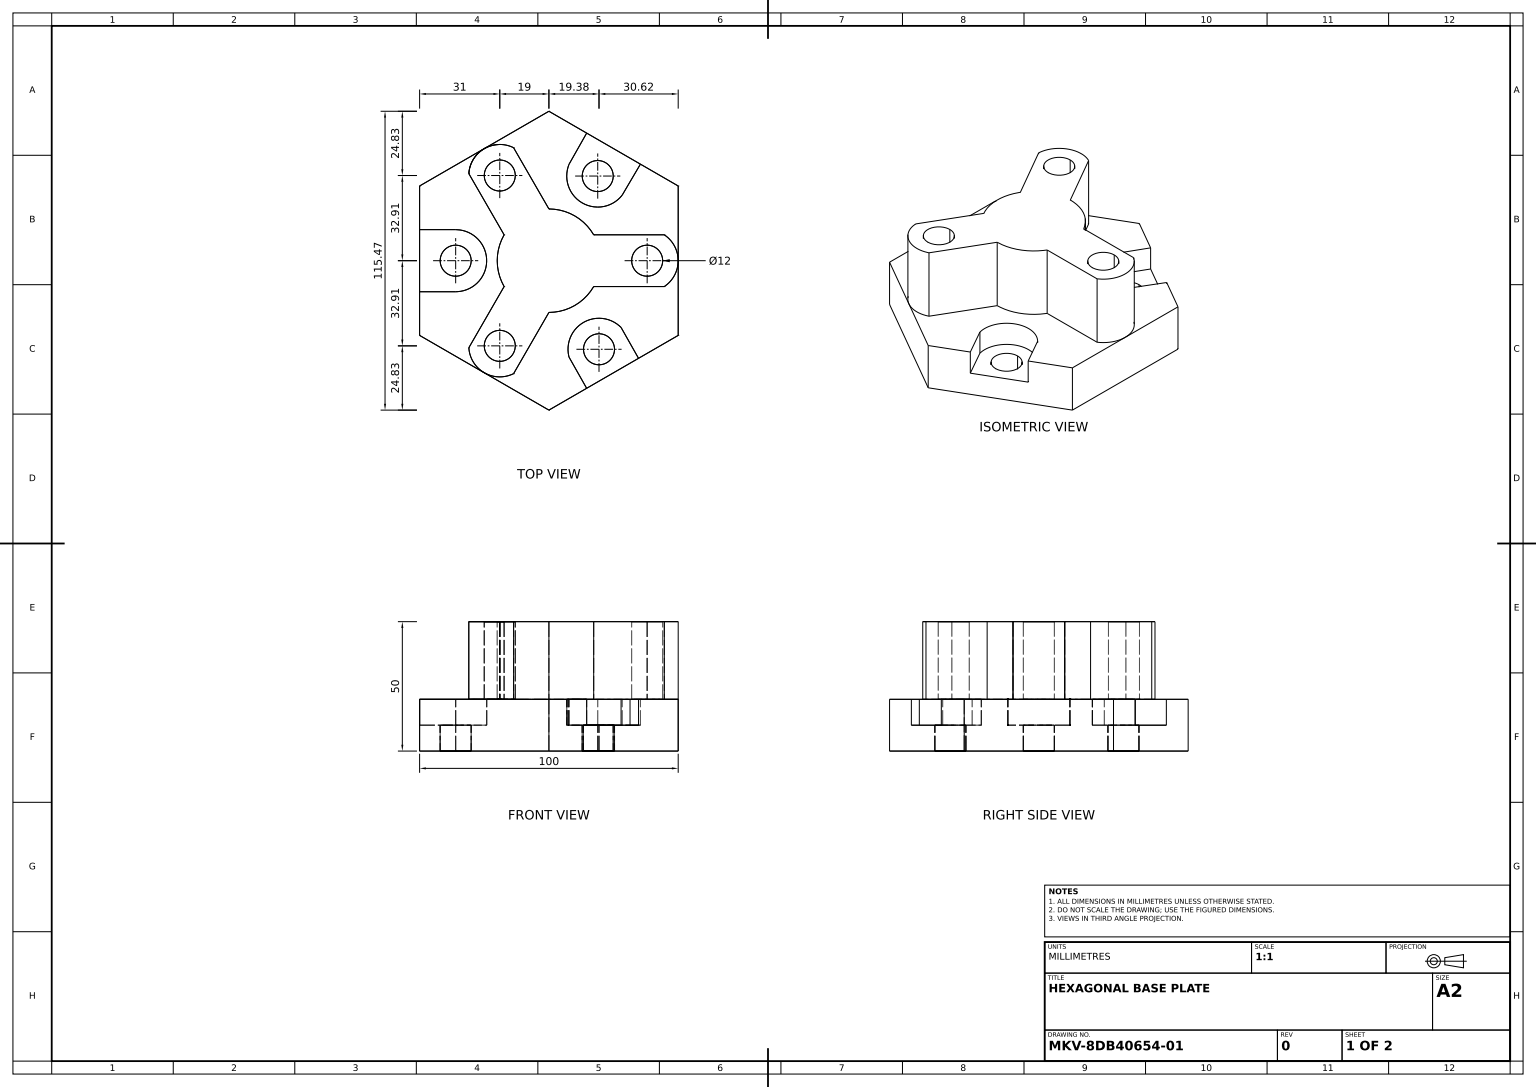
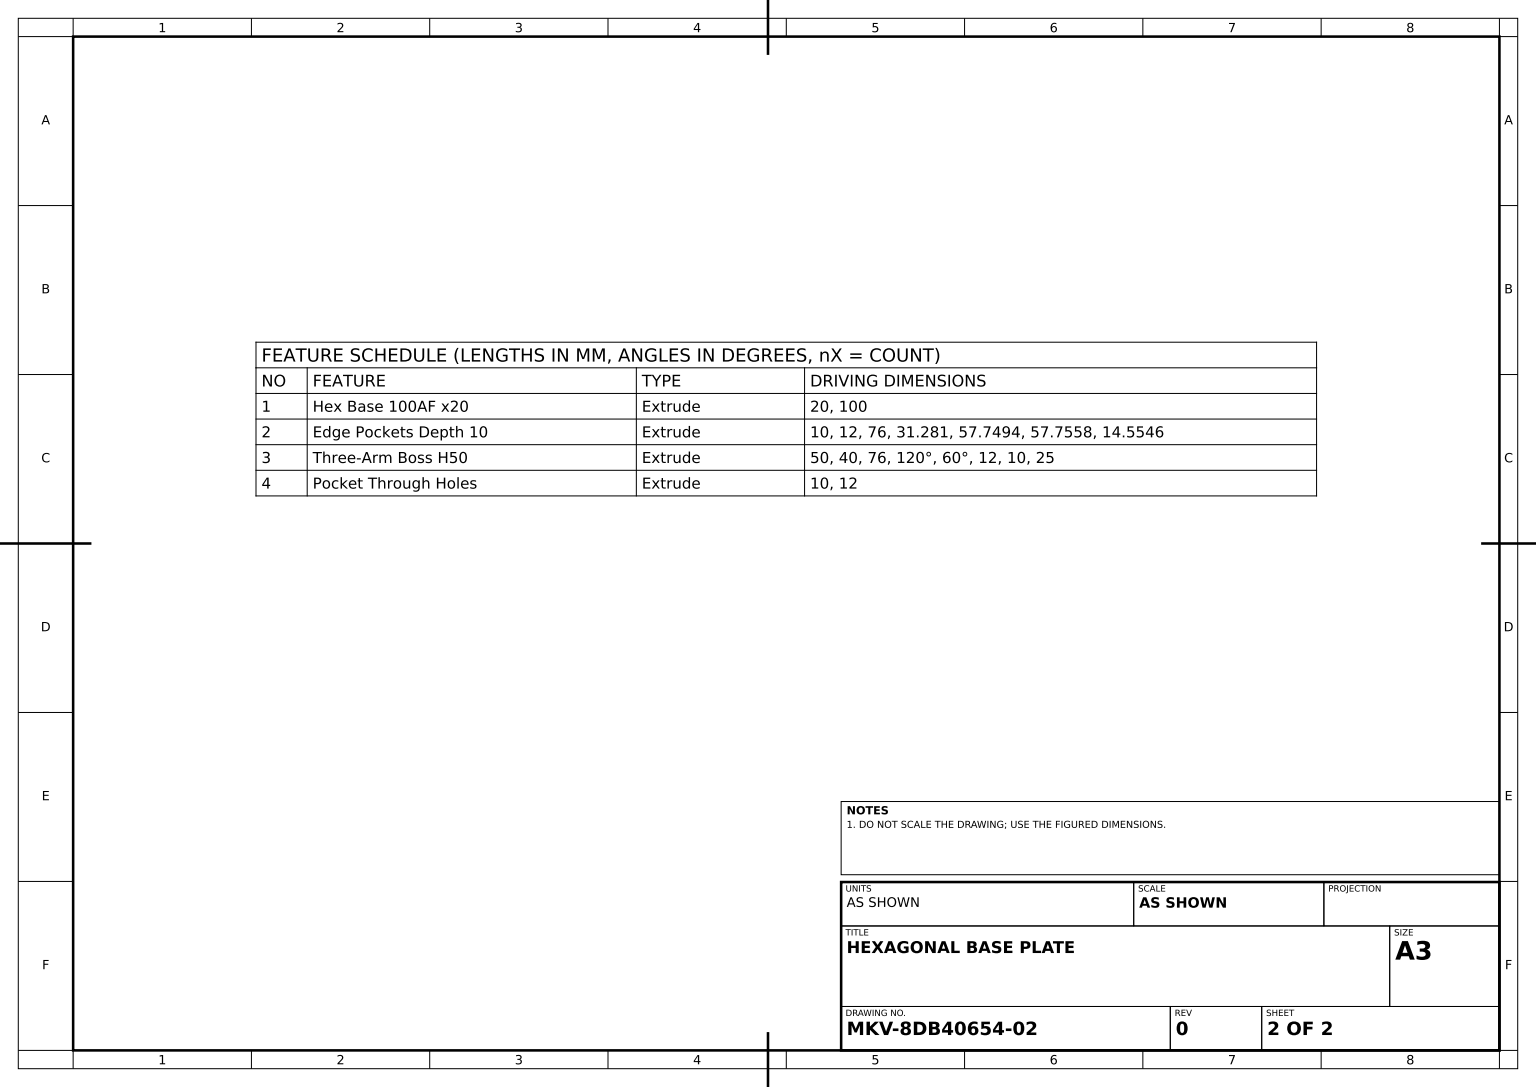
ISO-10303-21;
HEADER;
FILE_DESCRIPTION((''),'2;1');
FILE_NAME('','',(''),(''),'','','');
FILE_SCHEMA(('AUTOMOTIVE_DESIGN'));
ENDSEC;
DATA;
#1=APPLICATION_CONTEXT('');
#2=PRODUCT_CONTEXT('',#1,'mechanical');
#3=PRODUCT('','','',(#2));
#4=PRODUCT_DEFINITION_FORMATION('','',#3);
#5=PRODUCT_DEFINITION_CONTEXT('',#1,'design');
#6=PRODUCT_DEFINITION('','',#4,#5);
#7=PRODUCT_DEFINITION_SHAPE('','',#6);
#8=(LENGTH_UNIT()NAMED_UNIT(*)SI_UNIT(.MILLI.,.METRE.));
#9=(NAMED_UNIT(*)PLANE_ANGLE_UNIT()SI_UNIT($,.RADIAN.));
#10=(NAMED_UNIT(*)SI_UNIT($,.STERADIAN.)SOLID_ANGLE_UNIT());
#11=UNCERTAINTY_MEASURE_WITH_UNIT(LENGTH_MEASURE(1.E-05),#8,'distance_accuracy_value','');
#12=(GEOMETRIC_REPRESENTATION_CONTEXT(3)GLOBAL_UNCERTAINTY_ASSIGNED_CONTEXT((#11))GLOBAL_UNIT_ASSIGNED_CONTEXT((#8,#9,#10))REPRESENTATION_CONTEXT('',''));
#13=CARTESIAN_POINT('',(-50.,10.,-12.));
#14=VERTEX_POINT('',#13);
#15=CARTESIAN_POINT('',(-50.,20.,-12.));
#16=VERTEX_POINT('',#15);
#17=DIRECTION('',(0.,1.,0.));
#18=VECTOR('',#17,1000.);
#19=LINE('',#13,#18);
#20=EDGE_CURVE('',#14,#16,#19,.T.);
#21=ORIENTED_EDGE('',*,*,#20,.F.);
#22=CARTESIAN_POINT('',(-36.055514,10.,-12.));
#23=VERTEX_POINT('',#22);
#24=CARTESIAN_POINT('',(0.,10.,-12.));
#25=DIRECTION('',(1.,0.,0.));
#26=VECTOR('',#25,1000.);
#27=LINE('',#24,#26);
#28=EDGE_CURVE('',#14,#23,#27,.T.);
#29=ORIENTED_EDGE('',*,*,#28,.T.);
#30=CARTESIAN_POINT('',(-36.055514,20.,-12.));
#31=VERTEX_POINT('',#30);
#32=LINE('',#22,#18);
#33=EDGE_CURVE('',#23,#31,#32,.T.);
#34=ORIENTED_EDGE('',*,*,#33,.T.);
#35=CARTESIAN_POINT('',(0.,20.,-12.));
#36=LINE('',#35,#26);
#37=EDGE_CURVE('',#16,#31,#36,.T.);
#38=ORIENTED_EDGE('',*,*,#37,.F.);
#39=EDGE_LOOP('',(#21,#29,#34,#38));
#40=FACE_OUTER_BOUND('',#39,.T.);
#41=DIRECTION('',(0.,0.,1.));
#42=AXIS2_PLACEMENT_3D('',#24,#41,#25);
#43=PLANE('',#42);
#44=ADVANCED_FACE('',(#40),#43,.T.);
#45=CARTESIAN_POINT('',(18.881704,0.,-38.704071));
#46=VERTEX_POINT('',#45);
#47=CARTESIAN_POINT('',(18.881704,10.,-38.704071));
#48=VERTEX_POINT('',#47);
#49=LINE('',#45,#18);
#50=EDGE_CURVE('',#46,#48,#49,.T.);
#51=ORIENTED_EDGE('',*,*,#50,.F.);
#52=CARTESIAN_POINT('',(18.881704,0.,-26.704071));
#53=VERTEX_POINT('',#52);
#54=CARTESIAN_POINT('',(18.881704,0.,-32.704071));
#55=AXIS2_PLACEMENT_3D('',#54,#17,#41);
#56=CIRCLE('',#55,6.);
#57=EDGE_CURVE('',#53,#46,#56,.T.);
#58=ORIENTED_EDGE('',*,*,#57,.F.);
#59=CARTESIAN_POINT('',(18.881704,10.,-26.704071));
#60=VERTEX_POINT('',#59);
#61=LINE('',#52,#18);
#62=EDGE_CURVE('',#53,#60,#61,.T.);
#63=ORIENTED_EDGE('',*,*,#62,.T.);
#64=CARTESIAN_POINT('',(18.881704,10.,-32.704071));
#65=AXIS2_PLACEMENT_3D('',#64,#17,#41);
#66=CIRCLE('',#65,6.);
#67=EDGE_CURVE('',#60,#48,#66,.T.);
#68=ORIENTED_EDGE('',*,*,#67,.T.);
#69=EDGE_LOOP('',(#51,#58,#63,#68));
#70=FACE_OUTER_BOUND('',#69,.T.);
#71=CYLINDRICAL_SURFACE('',#55,6.);
#72=ADVANCED_FACE('',(#70),#71,.F.);
#73=CARTESIAN_POINT('',(50.,20.,0.));
#74=VERTEX_POINT('',#73);
#75=CARTESIAN_POINT('',(44.63325,20.,10.));
#76=VERTEX_POINT('',#75);
#77=CARTESIAN_POINT('',(38.,20.,0.));
#78=DIRECTION('',(0.,-1.,0.));
#79=AXIS2_PLACEMENT_3D('',#77,#78,#41);
#80=CIRCLE('',#79,12.);
#81=EDGE_CURVE('',#74,#76,#80,.T.);
#82=ORIENTED_EDGE('',*,*,#81,.F.);
#83=CARTESIAN_POINT('',(44.63325,20.,-10.));
#84=VERTEX_POINT('',#83);
#85=EDGE_CURVE('',#84,#74,#80,.T.);
#86=ORIENTED_EDGE('',*,*,#85,.F.);
#87=CARTESIAN_POINT('',(44.63325,50.,-10.));
#88=VERTEX_POINT('',#87);
#89=VECTOR('',#78,1000.);
#90=LINE('',#87,#89);
#91=EDGE_CURVE('',#88,#84,#90,.T.);
#92=ORIENTED_EDGE('',*,*,#91,.F.);
#93=CARTESIAN_POINT('',(44.63325,50.,10.));
#94=VERTEX_POINT('',#93);
#95=CARTESIAN_POINT('',(38.,50.,0.));
#96=AXIS2_PLACEMENT_3D('',#95,#17,#41);
#97=CIRCLE('',#96,12.);
#98=EDGE_CURVE('',#94,#88,#97,.T.);
#99=ORIENTED_EDGE('',*,*,#98,.F.);
#100=LINE('',#93,#89);
#101=EDGE_CURVE('',#94,#76,#100,.T.);
#102=ORIENTED_EDGE('',*,*,#101,.T.);
#103=EDGE_LOOP('',(#82,#86,#92,#99,#102));
#104=FACE_OUTER_BOUND('',#103,.T.);
#105=DIRECTION('',(0.,0.,-1.));
#106=AXIS2_PLACEMENT_3D('',#95,#78,#105);
#107=CYLINDRICAL_SURFACE('',#106,12.);
#108=ADVANCED_FACE('',(#104),#107,.T.);
#109=CARTESIAN_POINT('',(-36.055514,10.,12.));
#110=VERTEX_POINT('',#109);
#111=CARTESIAN_POINT('',(-36.055514,20.,12.));
#112=VERTEX_POINT('',#111);
#113=LINE('',#109,#18);
#114=EDGE_CURVE('',#110,#112,#113,.T.);
#115=ORIENTED_EDGE('',*,*,#114,.T.);
#116=CARTESIAN_POINT('',(-36.055514,20.,0.));
#117=AXIS2_PLACEMENT_3D('',#116,#78,#41);
#118=CIRCLE('',#117,12.);
#119=EDGE_CURVE('',#31,#112,#118,.T.);
#120=ORIENTED_EDGE('',*,*,#119,.F.);
#121=ORIENTED_EDGE('',*,*,#33,.F.);
#122=CARTESIAN_POINT('',(-36.055514,10.,0.));
#123=AXIS2_PLACEMENT_3D('',#122,#78,#41);
#124=CIRCLE('',#123,12.);
#125=EDGE_CURVE('',#23,#110,#124,.T.);
#126=ORIENTED_EDGE('',*,*,#125,.T.);
#127=EDGE_LOOP('',(#115,#120,#121,#126));
#128=FACE_OUTER_BOUND('',#127,.T.);
#129=AXIS2_PLACEMENT_3D('',#122,#17,#41);
#130=CYLINDRICAL_SURFACE('',#129,12.);
#131=ADVANCED_FACE('',(#128),#130,.F.);
#132=CARTESIAN_POINT('',(28.338333,20.,-25.316773));
#133=VERTEX_POINT('',#132);
#134=CARTESIAN_POINT('',(18.881704,20.,-20.704071));
#135=VERTEX_POINT('',#134);
#136=CARTESIAN_POINT('',(18.881704,20.,-32.704071));
#137=AXIS2_PLACEMENT_3D('',#136,#78,#41);
#138=CIRCLE('',#137,12.);
#139=EDGE_CURVE('',#133,#135,#138,.T.);
#140=ORIENTED_EDGE('',*,*,#139,.F.);
#141=CARTESIAN_POINT('',(28.338333,10.,-25.316773));
#142=VERTEX_POINT('',#141);
#143=LINE('',#141,#18);
#144=EDGE_CURVE('',#142,#133,#143,.T.);
#145=ORIENTED_EDGE('',*,*,#144,.F.);
#146=CARTESIAN_POINT('',(18.881704,10.,-20.704071));
#147=VERTEX_POINT('',#146);
#148=AXIS2_PLACEMENT_3D('',#64,#78,#41);
#149=CIRCLE('',#148,12.);
#150=EDGE_CURVE('',#142,#147,#149,.T.);
#151=ORIENTED_EDGE('',*,*,#150,.T.);
#152=LINE('',#146,#18);
#153=EDGE_CURVE('',#147,#135,#152,.T.);
#154=ORIENTED_EDGE('',*,*,#153,.T.);
#155=EDGE_LOOP('',(#140,#145,#151,#154));
#156=FACE_OUTER_BOUND('',#155,.T.);
#157=CYLINDRICAL_SURFACE('',#65,12.);
#158=ADVANCED_FACE('',(#156),#157,.F.);
#159=ORIENTED_EDGE('',*,*,#20,.T.);
#160=CARTESIAN_POINT('',(-50.,20.,-28.867513));
#161=VERTEX_POINT('',#160);
#162=VECTOR('',#41,1000.);
#163=LINE('',#160,#162);
#164=EDGE_CURVE('',#161,#16,#163,.T.);
#165=ORIENTED_EDGE('',*,*,#164,.F.);
#166=CARTESIAN_POINT('',(-50.,0.,-28.867513));
#167=VERTEX_POINT('',#166);
#168=LINE('',#160,#89);
#169=EDGE_CURVE('',#161,#167,#168,.T.);
#170=ORIENTED_EDGE('',*,*,#169,.T.);
#171=CARTESIAN_POINT('',(-50.,0.,28.867513));
#172=VERTEX_POINT('',#171);
#173=LINE('',#166,#162);
#174=EDGE_CURVE('',#167,#172,#173,.T.);
#175=ORIENTED_EDGE('',*,*,#174,.T.);
#176=CARTESIAN_POINT('',(-50.,20.,28.867513));
#177=VERTEX_POINT('',#176);
#178=LINE('',#176,#89);
#179=EDGE_CURVE('',#177,#172,#178,.T.);
#180=ORIENTED_EDGE('',*,*,#179,.F.);
#181=CARTESIAN_POINT('',(-50.,20.,12.));
#182=VERTEX_POINT('',#181);
#183=EDGE_CURVE('',#182,#177,#163,.T.);
#184=ORIENTED_EDGE('',*,*,#183,.F.);
#185=CARTESIAN_POINT('',(-50.,10.,12.));
#186=VERTEX_POINT('',#185);
#187=LINE('',#185,#18);
#188=EDGE_CURVE('',#186,#182,#187,.T.);
#189=ORIENTED_EDGE('',*,*,#188,.F.);
#190=CARTESIAN_POINT('',(-50.,10.,0.));
#191=LINE('',#190,#162);
#192=EDGE_CURVE('',#14,#186,#191,.T.);
#193=ORIENTED_EDGE('',*,*,#192,.F.);
#194=EDGE_LOOP('',(#159,#165,#170,#175,#180,#184,#189,#193));
#195=FACE_OUTER_BOUND('',#194,.T.);
#196=AXIS2_PLACEMENT_3D('',#160,#25,#105);
#197=PLANE('',#196);
#198=ADVANCED_FACE('',(#195),#197,.F.);
#199=CARTESIAN_POINT('',(-17.320508,50.,10.));
#200=VERTEX_POINT('',#199);
#201=CARTESIAN_POINT('',(-30.976879,50.,33.653528));
#202=VERTEX_POINT('',#201);
#203=CARTESIAN_POINT('',(-8.660254,50.,-5.));
#204=DIRECTION('',(-0.5,0.,0.866025404));
#205=VECTOR('',#204,1000.);
#206=LINE('',#203,#205);
#207=EDGE_CURVE('',#200,#202,#206,.T.);
#208=ORIENTED_EDGE('',*,*,#207,.T.);
#209=CARTESIAN_POINT('',(-13.656371,50.,43.653528));
#210=VERTEX_POINT('',#209);
#211=CARTESIAN_POINT('',(-19.,50.,32.908965));
#212=AXIS2_PLACEMENT_3D('',#211,#17,#41);
#213=CIRCLE('',#212,12.);
#214=EDGE_CURVE('',#202,#210,#213,.T.);
#215=ORIENTED_EDGE('',*,*,#214,.T.);
#216=CARTESIAN_POINT('',(0.,50.,20.));
#217=VERTEX_POINT('',#216);
#218=CARTESIAN_POINT('',(8.660254,50.,5.));
#219=LINE('',#218,#205);
#220=EDGE_CURVE('',#217,#210,#219,.T.);
#221=ORIENTED_EDGE('',*,*,#220,.F.);
#222=CARTESIAN_POINT('',(17.320508,50.,10.));
#223=VERTEX_POINT('',#222);
#224=CARTESIAN_POINT('',(0.,50.,0.));
#225=AXIS2_PLACEMENT_3D('',#224,#17,#41);
#226=CIRCLE('',#225,20.);
#227=EDGE_CURVE('',#217,#223,#226,.T.);
#228=ORIENTED_EDGE('',*,*,#227,.T.);
#229=CARTESIAN_POINT('',(0.,50.,10.));
#230=LINE('',#229,#26);
#231=EDGE_CURVE('',#223,#94,#230,.T.);
#232=ORIENTED_EDGE('',*,*,#231,.T.);
#233=ORIENTED_EDGE('',*,*,#98,.T.);
#234=CARTESIAN_POINT('',(17.320508,50.,-10.));
#235=VERTEX_POINT('',#234);
#236=CARTESIAN_POINT('',(0.,50.,-10.));
#237=LINE('',#236,#26);
#238=EDGE_CURVE('',#235,#88,#237,.T.);
#239=ORIENTED_EDGE('',*,*,#238,.F.);
#240=CARTESIAN_POINT('',(0.,50.,-20.));
#241=VERTEX_POINT('',#240);
#242=EDGE_CURVE('',#235,#241,#226,.T.);
#243=ORIENTED_EDGE('',*,*,#242,.T.);
#244=CARTESIAN_POINT('',(-13.656371,50.,-43.653528));
#245=VERTEX_POINT('',#244);
#246=CARTESIAN_POINT('',(8.660254,50.,-5.));
#247=DIRECTION('',(-0.5,0.,-0.866025404));
#248=VECTOR('',#247,1000.);
#249=LINE('',#246,#248);
#250=EDGE_CURVE('',#241,#245,#249,.T.);
#251=ORIENTED_EDGE('',*,*,#250,.T.);
#252=CARTESIAN_POINT('',(-19.,50.,-44.908965));
#253=VERTEX_POINT('',#252);
#254=CARTESIAN_POINT('',(-19.,50.,-32.908965));
#255=AXIS2_PLACEMENT_3D('',#254,#17,#41);
#256=CIRCLE('',#255,12.);
#257=EDGE_CURVE('',#245,#253,#256,.T.);
#258=ORIENTED_EDGE('',*,*,#257,.T.);
#259=CARTESIAN_POINT('',(-30.976879,50.,-33.653528));
#260=VERTEX_POINT('',#259);
#261=EDGE_CURVE('',#253,#260,#256,.T.);
#262=ORIENTED_EDGE('',*,*,#261,.T.);
#263=CARTESIAN_POINT('',(-17.320508,50.,-10.));
#264=VERTEX_POINT('',#263);
#265=CARTESIAN_POINT('',(-8.660254,50.,5.));
#266=LINE('',#265,#248);
#267=EDGE_CURVE('',#264,#260,#266,.T.);
#268=ORIENTED_EDGE('',*,*,#267,.F.);
#269=EDGE_CURVE('',#264,#200,#226,.T.);
#270=ORIENTED_EDGE('',*,*,#269,.T.);
#271=EDGE_LOOP('',(#208,#215,#221,#228,#232,#233,#239,#243,#251,#258,#262,#268,#270));
#272=FACE_OUTER_BOUND('',#271,.T.);
#273=CARTESIAN_POINT('',(-19.,50.,-38.908965));
#274=VERTEX_POINT('',#273);
#275=CARTESIAN_POINT('',(-19.,50.,-26.908965));
#276=VERTEX_POINT('',#275);
#277=CIRCLE('',#255,6.);
#278=EDGE_CURVE('',#274,#276,#277,.T.);
#279=ORIENTED_EDGE('',*,*,#278,.F.);
#280=EDGE_CURVE('',#276,#274,#277,.T.);
#281=ORIENTED_EDGE('',*,*,#280,.F.);
#282=EDGE_LOOP('',(#279,#281));
#283=FACE_BOUND('',#282,.T.);
#284=CARTESIAN_POINT('',(-19.,50.,38.908965));
#285=VERTEX_POINT('',#284);
#286=CARTESIAN_POINT('',(-19.,50.,26.908965));
#287=VERTEX_POINT('',#286);
#288=CIRCLE('',#212,6.);
#289=EDGE_CURVE('',#285,#287,#288,.T.);
#290=ORIENTED_EDGE('',*,*,#289,.F.);
#291=EDGE_CURVE('',#287,#285,#288,.T.);
#292=ORIENTED_EDGE('',*,*,#291,.F.);
#293=EDGE_LOOP('',(#290,#292));
#294=FACE_BOUND('',#293,.T.);
#295=CARTESIAN_POINT('',(38.,50.,6.));
#296=VERTEX_POINT('',#295);
#297=CARTESIAN_POINT('',(38.,50.,-6.));
#298=VERTEX_POINT('',#297);
#299=CIRCLE('',#96,6.);
#300=EDGE_CURVE('',#296,#298,#299,.T.);
#301=ORIENTED_EDGE('',*,*,#300,.F.);
#302=EDGE_CURVE('',#298,#296,#299,.T.);
#303=ORIENTED_EDGE('',*,*,#302,.F.);
#304=EDGE_LOOP('',(#301,#303));
#305=FACE_BOUND('',#304,.T.);
#306=PLANE('',#225);
#307=ADVANCED_FACE('',(#272,#283,#294,#305),#306,.T.);
#308=CARTESIAN_POINT('',(35.392305,10.,-37.30127));
#309=VERTEX_POINT('',#308);
#310=CARTESIAN_POINT('',(35.392305,20.,-37.30127));
#311=VERTEX_POINT('',#310);
#312=LINE('',#308,#18);
#313=EDGE_CURVE('',#309,#311,#312,.T.);
#314=ORIENTED_EDGE('',*,*,#313,.F.);
#315=CARTESIAN_POINT('',(9.979724,10.,5.87398));
#316=DIRECTION('',(-0.507248105,0.,0.86180007));
#317=VECTOR('',#316,1000.);
#318=LINE('',#315,#317);
#319=EDGE_CURVE('',#309,#142,#318,.T.);
#320=ORIENTED_EDGE('',*,*,#319,.T.);
#321=ORIENTED_EDGE('',*,*,#144,.T.);
#322=CARTESIAN_POINT('',(9.979724,20.,5.87398));
#323=LINE('',#322,#317);
#324=EDGE_CURVE('',#311,#133,#323,.T.);
#325=ORIENTED_EDGE('',*,*,#324,.F.);
#326=EDGE_LOOP('',(#314,#320,#321,#325));
#327=FACE_OUTER_BOUND('',#326,.T.);
#328=DIRECTION('',(-0.86180007,0.,-0.507248105));
#329=AXIS2_PLACEMENT_3D('',#315,#328,#316);
#330=PLANE('',#329);
#331=ADVANCED_FACE('',(#327),#330,.T.);
#332=CARTESIAN_POINT('',(-19.,20.,38.908965));
#333=VERTEX_POINT('',#332);
#334=CARTESIAN_POINT('',(-19.,20.,26.908965));
#335=VERTEX_POINT('',#334);
#336=CARTESIAN_POINT('',(-19.,20.,32.908965));
#337=AXIS2_PLACEMENT_3D('',#336,#78,#41);
#338=CIRCLE('',#337,6.);
#339=EDGE_CURVE('',#333,#335,#338,.T.);
#340=ORIENTED_EDGE('',*,*,#339,.F.);
#341=EDGE_CURVE('',#335,#333,#338,.T.);
#342=ORIENTED_EDGE('',*,*,#341,.F.);
#343=EDGE_LOOP('',(#340,#342));
#344=FACE_OUTER_BOUND('',#343,.T.);
#345=CARTESIAN_POINT('',(0.,20.,0.));
#346=AXIS2_PLACEMENT_3D('',#345,#17,#41);
#347=PLANE('',#346);
#348=ADVANCED_FACE('',(#344),#347,.T.);
#349=EDGE_CURVE('',#48,#60,#66,.T.);
#350=ORIENTED_EDGE('',*,*,#349,.T.);
#351=ORIENTED_EDGE('',*,*,#62,.F.);
#352=EDGE_CURVE('',#46,#53,#56,.T.);
#353=ORIENTED_EDGE('',*,*,#352,.F.);
#354=ORIENTED_EDGE('',*,*,#50,.T.);
#355=EDGE_LOOP('',(#350,#351,#353,#354));
#356=FACE_OUTER_BOUND('',#355,.T.);
#357=ADVANCED_FACE('',(#356),#71,.F.);
#358=CARTESIAN_POINT('',(19.375597,10.,40.229653));
#359=VERTEX_POINT('',#358);
#360=CARTESIAN_POINT('',(19.375597,10.,28.229653));
#361=VERTEX_POINT('',#360);
#362=CARTESIAN_POINT('',(19.375597,10.,34.229653));
#363=AXIS2_PLACEMENT_3D('',#362,#17,#41);
#364=CIRCLE('',#363,6.);
#365=EDGE_CURVE('',#359,#361,#364,.T.);
#366=ORIENTED_EDGE('',*,*,#365,.T.);
#367=CARTESIAN_POINT('',(19.375597,0.,28.229653));
#368=VERTEX_POINT('',#367);
#369=LINE('',#367,#18);
#370=EDGE_CURVE('',#368,#361,#369,.T.);
#371=ORIENTED_EDGE('',*,*,#370,.F.);
#372=CARTESIAN_POINT('',(19.375597,0.,40.229653));
#373=VERTEX_POINT('',#372);
#374=CARTESIAN_POINT('',(19.375597,0.,34.229653));
#375=AXIS2_PLACEMENT_3D('',#374,#17,#41);
#376=CIRCLE('',#375,6.);
#377=EDGE_CURVE('',#373,#368,#376,.T.);
#378=ORIENTED_EDGE('',*,*,#377,.F.);
#379=LINE('',#372,#18);
#380=EDGE_CURVE('',#373,#359,#379,.T.);
#381=ORIENTED_EDGE('',*,*,#380,.T.);
#382=EDGE_LOOP('',(#366,#371,#378,#381));
#383=FACE_OUTER_BOUND('',#382,.T.);
#384=CYLINDRICAL_SURFACE('',#375,6.);
#385=ADVANCED_FACE('',(#383),#384,.F.);
#386=CARTESIAN_POINT('',(17.320508,20.,10.));
#387=VERTEX_POINT('',#386);
#388=CARTESIAN_POINT('',(0.,20.,20.));
#389=VERTEX_POINT('',#388);
#390=AXIS2_PLACEMENT_3D('',#345,#78,#41);
#391=CIRCLE('',#390,20.);
#392=EDGE_CURVE('',#387,#389,#391,.T.);
#393=ORIENTED_EDGE('',*,*,#392,.F.);
#394=LINE('',#222,#89);
#395=EDGE_CURVE('',#223,#387,#394,.T.);
#396=ORIENTED_EDGE('',*,*,#395,.F.);
#397=ORIENTED_EDGE('',*,*,#227,.F.);
#398=LINE('',#216,#89);
#399=EDGE_CURVE('',#217,#389,#398,.T.);
#400=ORIENTED_EDGE('',*,*,#399,.T.);
#401=EDGE_LOOP('',(#393,#396,#397,#400));
#402=FACE_OUTER_BOUND('',#401,.T.);
#403=AXIS2_PLACEMENT_3D('',#224,#78,#105);
#404=CYLINDRICAL_SURFACE('',#403,20.);
#405=ADVANCED_FACE('',(#402),#404,.T.);
#406=CARTESIAN_POINT('',(14.600746,20.,49.305283));
#407=VERTEX_POINT('',#406);
#408=CARTESIAN_POINT('',(7.749398,20.,37.201437));
#409=VERTEX_POINT('',#408);
#410=CARTESIAN_POINT('',(-10.078972,20.,5.705173));
#411=DIRECTION('',(-0.49260442,0.,-0.870253346));
#412=VECTOR('',#411,1000.);
#413=LINE('',#410,#412);
#414=EDGE_CURVE('',#407,#409,#413,.T.);
#415=ORIENTED_EDGE('',*,*,#414,.F.);
#416=CARTESIAN_POINT('',(14.600746,10.,49.305283));
#417=VERTEX_POINT('',#416);
#418=LINE('',#416,#18);
#419=EDGE_CURVE('',#417,#407,#418,.T.);
#420=ORIENTED_EDGE('',*,*,#419,.F.);
#421=CARTESIAN_POINT('',(7.749398,10.,37.201437));
#422=VERTEX_POINT('',#421);
#423=CARTESIAN_POINT('',(-10.078972,10.,5.705173));
#424=LINE('',#423,#412);
#425=EDGE_CURVE('',#417,#422,#424,.T.);
#426=ORIENTED_EDGE('',*,*,#425,.T.);
#427=LINE('',#421,#18);
#428=EDGE_CURVE('',#422,#409,#427,.T.);
#429=ORIENTED_EDGE('',*,*,#428,.T.);
#430=EDGE_LOOP('',(#415,#420,#426,#429));
#431=FACE_OUTER_BOUND('',#430,.T.);
#432=DIRECTION('',(0.870253346,0.,-0.49260442));
#433=AXIS2_PLACEMENT_3D('',#423,#432,#411);
#434=PLANE('',#433);
#435=ADVANCED_FACE('',(#431),#434,.T.);
#436=CARTESIAN_POINT('',(-30.976879,20.,-33.653528));
#437=VERTEX_POINT('',#436);
#438=LINE('',#259,#89);
#439=EDGE_CURVE('',#260,#437,#438,.T.);
#440=ORIENTED_EDGE('',*,*,#439,.T.);
#441=CARTESIAN_POINT('',(-17.320508,20.,-10.));
#442=VERTEX_POINT('',#441);
#443=CARTESIAN_POINT('',(-8.660254,20.,5.));
#444=DIRECTION('',(0.5,0.,0.866025404));
#445=VECTOR('',#444,1000.);
#446=LINE('',#443,#445);
#447=EDGE_CURVE('',#437,#442,#446,.T.);
#448=ORIENTED_EDGE('',*,*,#447,.T.);
#449=LINE('',#263,#89);
#450=EDGE_CURVE('',#264,#442,#449,.T.);
#451=ORIENTED_EDGE('',*,*,#450,.F.);
#452=ORIENTED_EDGE('',*,*,#267,.T.);
#453=EDGE_LOOP('',(#440,#448,#451,#452));
#454=FACE_OUTER_BOUND('',#453,.T.);
#455=DIRECTION('',(-0.866025404,0.,0.5));
#456=AXIS2_PLACEMENT_3D('',#265,#455,#444);
#457=PLANE('',#456);
#458=ADVANCED_FACE('',(#454),#457,.T.);
#459=CARTESIAN_POINT('',(38.,20.,6.));
#460=VERTEX_POINT('',#459);
#461=CARTESIAN_POINT('',(38.,20.,-6.));
#462=VERTEX_POINT('',#461);
#463=CIRCLE('',#79,6.);
#464=EDGE_CURVE('',#460,#462,#463,.T.);
#465=ORIENTED_EDGE('',*,*,#464,.T.);
#466=LINE('',#297,#89);
#467=EDGE_CURVE('',#298,#462,#466,.T.);
#468=ORIENTED_EDGE('',*,*,#467,.F.);
#469=ORIENTED_EDGE('',*,*,#302,.T.);
#470=LINE('',#295,#89);
#471=EDGE_CURVE('',#296,#460,#470,.T.);
#472=ORIENTED_EDGE('',*,*,#471,.T.);
#473=EDGE_LOOP('',(#465,#468,#469,#472));
#474=FACE_OUTER_BOUND('',#473,.T.);
#475=CYLINDRICAL_SURFACE('',#106,6.);
#476=ADVANCED_FACE('',(#474),#475,.F.);
#477=ORIENTED_EDGE('',*,*,#238,.T.);
#478=ORIENTED_EDGE('',*,*,#91,.T.);
#479=CARTESIAN_POINT('',(17.320508,20.,-10.));
#480=VERTEX_POINT('',#479);
#481=CARTESIAN_POINT('',(0.,20.,-10.));
#482=DIRECTION('',(-1.,0.,0.));
#483=VECTOR('',#482,1000.);
#484=LINE('',#481,#483);
#485=EDGE_CURVE('',#84,#480,#484,.T.);
#486=ORIENTED_EDGE('',*,*,#485,.T.);
#487=LINE('',#234,#89);
#488=EDGE_CURVE('',#235,#480,#487,.T.);
#489=ORIENTED_EDGE('',*,*,#488,.F.);
#490=EDGE_LOOP('',(#477,#478,#486,#489));
#491=FACE_OUTER_BOUND('',#490,.T.);
#492=AXIS2_PLACEMENT_3D('',#236,#105,#482);
#493=PLANE('',#492);
#494=ADVANCED_FACE('',(#491),#493,.T.);
#495=ORIENTED_EDGE('',*,*,#341,.T.);
#496=LINE('',#284,#89);
#497=EDGE_CURVE('',#285,#333,#496,.T.);
#498=ORIENTED_EDGE('',*,*,#497,.F.);
#499=ORIENTED_EDGE('',*,*,#289,.T.);
#500=LINE('',#286,#89);
#501=EDGE_CURVE('',#287,#335,#500,.T.);
#502=ORIENTED_EDGE('',*,*,#501,.T.);
#503=EDGE_LOOP('',(#495,#498,#499,#502));
#504=FACE_OUTER_BOUND('',#503,.T.);
#505=AXIS2_PLACEMENT_3D('',#211,#78,#105);
#506=CYLINDRICAL_SURFACE('',#505,6.);
#507=ADVANCED_FACE('',(#504),#506,.F.);
#508=ORIENTED_EDGE('',*,*,#261,.F.);
#509=CARTESIAN_POINT('',(-19.,20.,-44.908965));
#510=VERTEX_POINT('',#509);
#511=LINE('',#252,#89);
#512=EDGE_CURVE('',#253,#510,#511,.T.);
#513=ORIENTED_EDGE('',*,*,#512,.T.);
#514=CARTESIAN_POINT('',(-25.,20.,-43.30127));
#515=VERTEX_POINT('',#514);
#516=CARTESIAN_POINT('',(-19.,20.,-32.908965));
#517=AXIS2_PLACEMENT_3D('',#516,#78,#41);
#518=CIRCLE('',#517,12.);
#519=EDGE_CURVE('',#515,#510,#518,.T.);
#520=ORIENTED_EDGE('',*,*,#519,.F.);
#521=EDGE_CURVE('',#437,#515,#518,.T.);
#522=ORIENTED_EDGE('',*,*,#521,.F.);
#523=ORIENTED_EDGE('',*,*,#439,.F.);
#524=EDGE_LOOP('',(#508,#513,#520,#522,#523));
#525=FACE_OUTER_BOUND('',#524,.T.);
#526=AXIS2_PLACEMENT_3D('',#254,#78,#105);
#527=CYLINDRICAL_SURFACE('',#526,12.);
#528=ADVANCED_FACE('',(#525),#527,.T.);
#529=CARTESIAN_POINT('',(-17.320508,20.,10.));
#530=VERTEX_POINT('',#529);
#531=LINE('',#199,#89);
#532=EDGE_CURVE('',#200,#530,#531,.T.);
#533=ORIENTED_EDGE('',*,*,#532,.F.);
#534=ORIENTED_EDGE('',*,*,#269,.F.);
#535=ORIENTED_EDGE('',*,*,#450,.T.);
#536=EDGE_CURVE('',#530,#442,#391,.T.);
#537=ORIENTED_EDGE('',*,*,#536,.F.);
#538=EDGE_LOOP('',(#533,#534,#535,#537));
#539=FACE_OUTER_BOUND('',#538,.T.);
#540=ADVANCED_FACE('',(#539),#404,.T.);
#541=ORIENTED_EDGE('',*,*,#242,.F.);
#542=ORIENTED_EDGE('',*,*,#488,.T.);
#543=CARTESIAN_POINT('',(0.,20.,-20.));
#544=VERTEX_POINT('',#543);
#545=EDGE_CURVE('',#544,#480,#391,.T.);
#546=ORIENTED_EDGE('',*,*,#545,.F.);
#547=LINE('',#240,#89);
#548=EDGE_CURVE('',#241,#544,#547,.T.);
#549=ORIENTED_EDGE('',*,*,#548,.F.);
#550=EDGE_LOOP('',(#541,#542,#546,#549));
#551=FACE_OUTER_BOUND('',#550,.T.);
#552=ADVANCED_FACE('',(#551),#404,.T.);
#553=ORIENTED_EDGE('',*,*,#419,.T.);
#554=CARTESIAN_POINT('',(0.,20.,57.735027));
#555=VERTEX_POINT('',#554);
#556=DIRECTION('',(0.866025404,0.,-0.5));
#557=VECTOR('',#556,1000.);
#558=LINE('',#554,#557);
#559=EDGE_CURVE('',#555,#407,#558,.T.);
#560=ORIENTED_EDGE('',*,*,#559,.F.);
#561=CARTESIAN_POINT('',(0.,0.,57.735027));
#562=VERTEX_POINT('',#561);
#563=LINE('',#554,#89);
#564=EDGE_CURVE('',#555,#562,#563,.T.);
#565=ORIENTED_EDGE('',*,*,#564,.T.);
#566=CARTESIAN_POINT('',(50.,0.,28.867513));
#567=VERTEX_POINT('',#566);
#568=LINE('',#561,#557);
#569=EDGE_CURVE('',#562,#567,#568,.T.);
#570=ORIENTED_EDGE('',*,*,#569,.T.);
#571=CARTESIAN_POINT('',(50.,20.,28.867513));
#572=VERTEX_POINT('',#571);
#573=LINE('',#571,#89);
#574=EDGE_CURVE('',#572,#567,#573,.T.);
#575=ORIENTED_EDGE('',*,*,#574,.F.);
#576=CARTESIAN_POINT('',(34.661484,20.,37.72321));
#577=VERTEX_POINT('',#576);
#578=EDGE_CURVE('',#577,#572,#558,.T.);
#579=ORIENTED_EDGE('',*,*,#578,.F.);
#580=CARTESIAN_POINT('',(34.661484,10.,37.72321));
#581=VERTEX_POINT('',#580);
#582=LINE('',#580,#18);
#583=EDGE_CURVE('',#581,#577,#582,.T.);
#584=ORIENTED_EDGE('',*,*,#583,.F.);
#585=CARTESIAN_POINT('',(25.,10.,43.30127));
#586=LINE('',#585,#557);
#587=EDGE_CURVE('',#417,#581,#586,.T.);
#588=ORIENTED_EDGE('',*,*,#587,.F.);
#589=EDGE_LOOP('',(#553,#560,#565,#570,#575,#579,#584,#588));
#590=FACE_OUTER_BOUND('',#589,.T.);
#591=AXIS2_PLACEMENT_3D('',#554,#247,#455);
#592=PLANE('',#591);
#593=ADVANCED_FACE('',(#590),#592,.F.);
#594=CARTESIAN_POINT('',(7.755802,10.,-37.200103));
#595=VERTEX_POINT('',#594);
#596=EDGE_CURVE('',#147,#595,#149,.T.);
#597=ORIENTED_EDGE('',*,*,#596,.T.);
#598=CARTESIAN_POINT('',(7.755802,20.,-37.200103));
#599=VERTEX_POINT('',#598);
#600=LINE('',#594,#18);
#601=EDGE_CURVE('',#595,#599,#600,.T.);
#602=ORIENTED_EDGE('',*,*,#601,.T.);
#603=EDGE_CURVE('',#135,#599,#138,.T.);
#604=ORIENTED_EDGE('',*,*,#603,.F.);
#605=ORIENTED_EDGE('',*,*,#153,.F.);
#606=EDGE_LOOP('',(#597,#602,#604,#605));
#607=FACE_OUTER_BOUND('',#606,.T.);
#608=ADVANCED_FACE('',(#607),#157,.F.);
#609=CARTESIAN_POINT('',(27.907342,10.,25.791091));
#610=VERTEX_POINT('',#609);
#611=CARTESIAN_POINT('',(27.907342,20.,25.791091));
#612=VERTEX_POINT('',#611);
#613=LINE('',#609,#18);
#614=EDGE_CURVE('',#610,#612,#613,.T.);
#615=ORIENTED_EDGE('',*,*,#614,.F.);
#616=CARTESIAN_POINT('',(10.078972,10.,-5.705173));
#617=DIRECTION('',(0.49260442,0.,0.870253346));
#618=VECTOR('',#617,1000.);
#619=LINE('',#616,#618);
#620=EDGE_CURVE('',#610,#581,#619,.T.);
#621=ORIENTED_EDGE('',*,*,#620,.T.);
#622=ORIENTED_EDGE('',*,*,#583,.T.);
#623=CARTESIAN_POINT('',(10.078972,20.,-5.705173));
#624=LINE('',#623,#618);
#625=EDGE_CURVE('',#612,#577,#624,.T.);
#626=ORIENTED_EDGE('',*,*,#625,.F.);
#627=EDGE_LOOP('',(#615,#621,#622,#626));
#628=FACE_OUTER_BOUND('',#627,.T.);
#629=DIRECTION('',(-0.870253346,0.,0.49260442));
#630=AXIS2_PLACEMENT_3D('',#616,#629,#617);
#631=PLANE('',#630);
#632=ADVANCED_FACE('',(#628),#631,.T.);
#633=CARTESIAN_POINT('',(14.607695,10.,-49.30127));
#634=VERTEX_POINT('',#633);
#635=CARTESIAN_POINT('',(-10.076878,10.,-5.705705));
#636=DIRECTION('',(-0.492716701,0.,0.87018978));
#637=VECTOR('',#636,1000.);
#638=LINE('',#635,#637);
#639=EDGE_CURVE('',#634,#595,#638,.T.);
#640=ORIENTED_EDGE('',*,*,#639,.F.);
#641=CARTESIAN_POINT('',(14.607695,20.,-49.30127));
#642=VERTEX_POINT('',#641);
#643=LINE('',#633,#18);
#644=EDGE_CURVE('',#634,#642,#643,.T.);
#645=ORIENTED_EDGE('',*,*,#644,.T.);
#646=CARTESIAN_POINT('',(-10.076878,20.,-5.705705));
#647=LINE('',#646,#637);
#648=EDGE_CURVE('',#642,#599,#647,.T.);
#649=ORIENTED_EDGE('',*,*,#648,.T.);
#650=ORIENTED_EDGE('',*,*,#601,.F.);
#651=EDGE_LOOP('',(#640,#645,#649,#650));
#652=FACE_OUTER_BOUND('',#651,.T.);
#653=DIRECTION('',(-0.87018978,0.,-0.492716701));
#654=AXIS2_PLACEMENT_3D('',#635,#653,#636);
#655=PLANE('',#654);
#656=ADVANCED_FACE('',(#652),#655,.F.);
#657=CARTESIAN_POINT('',(-36.055514,10.,-6.));
#658=VERTEX_POINT('',#657);
#659=CARTESIAN_POINT('',(-36.055514,10.,6.));
#660=VERTEX_POINT('',#659);
#661=CIRCLE('',#129,6.);
#662=EDGE_CURVE('',#658,#660,#661,.T.);
#663=ORIENTED_EDGE('',*,*,#662,.F.);
#664=EDGE_CURVE('',#660,#658,#661,.T.);
#665=ORIENTED_EDGE('',*,*,#664,.F.);
#666=EDGE_LOOP('',(#663,#665));
#667=FACE_BOUND('',#666,.T.);
#668=ORIENTED_EDGE('',*,*,#125,.F.);
#669=ORIENTED_EDGE('',*,*,#28,.F.);
#670=ORIENTED_EDGE('',*,*,#192,.T.);
#671=CARTESIAN_POINT('',(0.,10.,12.));
#672=LINE('',#671,#26);
#673=EDGE_CURVE('',#186,#110,#672,.T.);
#674=ORIENTED_EDGE('',*,*,#673,.T.);
#675=EDGE_LOOP('',(#668,#669,#670,#674));
#676=FACE_OUTER_BOUND('',#675,.T.);
#677=CARTESIAN_POINT('',(0.,10.,0.));
#678=AXIS2_PLACEMENT_3D('',#677,#17,#41);
#679=PLANE('',#678);
#680=ADVANCED_FACE('',(#667,#676),#679,.T.);
#681=ORIENTED_EDGE('',*,*,#214,.F.);
#682=CARTESIAN_POINT('',(-30.976879,20.,33.653528));
#683=VERTEX_POINT('',#682);
#684=LINE('',#201,#89);
#685=EDGE_CURVE('',#202,#683,#684,.T.);
#686=ORIENTED_EDGE('',*,*,#685,.T.);
#687=CARTESIAN_POINT('',(-25.,20.,43.30127));
#688=VERTEX_POINT('',#687);
#689=CIRCLE('',#337,12.);
#690=EDGE_CURVE('',#688,#683,#689,.T.);
#691=ORIENTED_EDGE('',*,*,#690,.F.);
#692=CARTESIAN_POINT('',(-13.656371,20.,43.653528));
#693=VERTEX_POINT('',#692);
#694=EDGE_CURVE('',#693,#688,#689,.T.);
#695=ORIENTED_EDGE('',*,*,#694,.F.);
#696=LINE('',#209,#89);
#697=EDGE_CURVE('',#210,#693,#696,.T.);
#698=ORIENTED_EDGE('',*,*,#697,.F.);
#699=EDGE_LOOP('',(#681,#686,#691,#695,#698));
#700=FACE_OUTER_BOUND('',#699,.T.);
#701=CYLINDRICAL_SURFACE('',#505,12.);
#702=ADVANCED_FACE('',(#700),#701,.T.);
#703=ORIENTED_EDGE('',*,*,#464,.F.);
#704=EDGE_CURVE('',#462,#460,#463,.T.);
#705=ORIENTED_EDGE('',*,*,#704,.F.);
#706=EDGE_LOOP('',(#703,#705));
#707=FACE_OUTER_BOUND('',#706,.T.);
#708=ADVANCED_FACE('',(#707),#347,.T.);
#709=CARTESIAN_POINT('',(8.660254,20.,5.));
#710=DIRECTION('',(0.5,0.,-0.866025404));
#711=VECTOR('',#710,1000.);
#712=LINE('',#709,#711);
#713=EDGE_CURVE('',#693,#389,#712,.T.);
#714=ORIENTED_EDGE('',*,*,#713,.T.);
#715=ORIENTED_EDGE('',*,*,#399,.F.);
#716=ORIENTED_EDGE('',*,*,#220,.T.);
#717=ORIENTED_EDGE('',*,*,#697,.T.);
#718=EDGE_LOOP('',(#714,#715,#716,#717));
#719=FACE_OUTER_BOUND('',#718,.T.);
#720=DIRECTION('',(0.866025404,0.,0.5));
#721=AXIS2_PLACEMENT_3D('',#218,#720,#710);
#722=PLANE('',#721);
#723=ADVANCED_FACE('',(#719),#722,.T.);
#724=VECTOR('',#720,1000.);
#725=LINE('',#176,#724);
#726=EDGE_CURVE('',#688,#555,#725,.T.);
#727=ORIENTED_EDGE('',*,*,#726,.F.);
#728=EDGE_CURVE('',#177,#688,#725,.T.);
#729=ORIENTED_EDGE('',*,*,#728,.F.);
#730=ORIENTED_EDGE('',*,*,#179,.T.);
#731=LINE('',#171,#724);
#732=EDGE_CURVE('',#172,#562,#731,.T.);
#733=ORIENTED_EDGE('',*,*,#732,.T.);
#734=ORIENTED_EDGE('',*,*,#564,.F.);
#735=EDGE_LOOP('',(#727,#729,#730,#733,#734));
#736=FACE_OUTER_BOUND('',#735,.T.);
#737=DIRECTION('',(-0.866025404,0.,-0.5));
#738=AXIS2_PLACEMENT_3D('',#176,#710,#737);
#739=PLANE('',#738);
#740=ADVANCED_FACE('',(#736),#739,.F.);
#741=ORIENTED_EDGE('',*,*,#625,.T.);
#742=ORIENTED_EDGE('',*,*,#578,.T.);
#743=VECTOR('',#105,1000.);
#744=LINE('',#571,#743);
#745=EDGE_CURVE('',#572,#74,#744,.T.);
#746=ORIENTED_EDGE('',*,*,#745,.T.);
#747=ORIENTED_EDGE('',*,*,#81,.T.);
#748=CARTESIAN_POINT('',(0.,20.,10.));
#749=LINE('',#748,#483);
#750=EDGE_CURVE('',#76,#387,#749,.T.);
#751=ORIENTED_EDGE('',*,*,#750,.T.);
#752=ORIENTED_EDGE('',*,*,#392,.T.);
#753=ORIENTED_EDGE('',*,*,#713,.F.);
#754=ORIENTED_EDGE('',*,*,#694,.T.);
#755=ORIENTED_EDGE('',*,*,#726,.T.);
#756=ORIENTED_EDGE('',*,*,#559,.T.);
#757=ORIENTED_EDGE('',*,*,#414,.T.);
#758=CARTESIAN_POINT('',(19.375597,20.,34.229653));
#759=AXIS2_PLACEMENT_3D('',#758,#78,#41);
#760=CIRCLE('',#759,12.);
#761=EDGE_CURVE('',#409,#612,#760,.T.);
#762=ORIENTED_EDGE('',*,*,#761,.T.);
#763=EDGE_LOOP('',(#741,#742,#746,#747,#751,#752,#753,#754,#755,#756,#757,#762));
#764=FACE_OUTER_BOUND('',#763,.T.);
#765=ADVANCED_FACE('',(#764),#347,.T.);
#766=ORIENTED_EDGE('',*,*,#536,.T.);
#767=ORIENTED_EDGE('',*,*,#447,.F.);
#768=ORIENTED_EDGE('',*,*,#521,.T.);
#769=CARTESIAN_POINT('',(0.,20.,-57.735027));
#770=VECTOR('',#455,1000.);
#771=LINE('',#769,#770);
#772=EDGE_CURVE('',#515,#161,#771,.T.);
#773=ORIENTED_EDGE('',*,*,#772,.T.);
#774=ORIENTED_EDGE('',*,*,#164,.T.);
#775=ORIENTED_EDGE('',*,*,#37,.T.);
#776=ORIENTED_EDGE('',*,*,#119,.T.);
#777=CARTESIAN_POINT('',(0.,20.,12.));
#778=LINE('',#777,#26);
#779=EDGE_CURVE('',#182,#112,#778,.T.);
#780=ORIENTED_EDGE('',*,*,#779,.F.);
#781=ORIENTED_EDGE('',*,*,#183,.T.);
#782=ORIENTED_EDGE('',*,*,#728,.T.);
#783=ORIENTED_EDGE('',*,*,#690,.T.);
#784=CARTESIAN_POINT('',(-8.660254,20.,-5.));
#785=LINE('',#784,#711);
#786=EDGE_CURVE('',#683,#530,#785,.T.);
#787=ORIENTED_EDGE('',*,*,#786,.T.);
#788=EDGE_LOOP('',(#766,#767,#768,#773,#774,#775,#776,#780,#781,#782,#783,#787));
#789=FACE_OUTER_BOUND('',#788,.T.);
#790=ADVANCED_FACE('',(#789),#347,.T.);
#791=ORIENTED_EDGE('',*,*,#278,.T.);
#792=CARTESIAN_POINT('',(-19.,20.,-26.908965));
#793=VERTEX_POINT('',#792);
#794=LINE('',#275,#89);
#795=EDGE_CURVE('',#276,#793,#794,.T.);
#796=ORIENTED_EDGE('',*,*,#795,.T.);
#797=CARTESIAN_POINT('',(-19.,20.,-38.908965));
#798=VERTEX_POINT('',#797);
#799=CIRCLE('',#517,6.);
#800=EDGE_CURVE('',#793,#798,#799,.T.);
#801=ORIENTED_EDGE('',*,*,#800,.T.);
#802=LINE('',#273,#89);
#803=EDGE_CURVE('',#274,#798,#802,.T.);
#804=ORIENTED_EDGE('',*,*,#803,.F.);
#805=EDGE_LOOP('',(#791,#796,#801,#804));
#806=FACE_OUTER_BOUND('',#805,.T.);
#807=CYLINDRICAL_SURFACE('',#526,6.);
#808=ADVANCED_FACE('',(#806),#807,.F.);
#809=ORIENTED_EDGE('',*,*,#548,.T.);
#810=CARTESIAN_POINT('',(-13.656371,20.,-43.653528));
#811=VERTEX_POINT('',#810);
#812=CARTESIAN_POINT('',(8.660254,20.,-5.));
#813=LINE('',#812,#445);
#814=EDGE_CURVE('',#811,#544,#813,.T.);
#815=ORIENTED_EDGE('',*,*,#814,.F.);
#816=LINE('',#244,#89);
#817=EDGE_CURVE('',#245,#811,#816,.T.);
#818=ORIENTED_EDGE('',*,*,#817,.F.);
#819=ORIENTED_EDGE('',*,*,#250,.F.);
#820=EDGE_LOOP('',(#809,#815,#818,#819));
#821=FACE_OUTER_BOUND('',#820,.T.);
#822=AXIS2_PLACEMENT_3D('',#246,#455,#444);
#823=PLANE('',#822);
#824=ADVANCED_FACE('',(#821),#823,.F.);
#825=VERTEX_POINT('',#769);
#826=CARTESIAN_POINT('',(0.,0.,-57.735027));
#827=VERTEX_POINT('',#826);
#828=LINE('',#769,#89);
#829=EDGE_CURVE('',#825,#827,#828,.T.);
#830=ORIENTED_EDGE('',*,*,#829,.F.);
#831=CARTESIAN_POINT('',(50.,20.,-28.867513));
#832=VECTOR('',#737,1000.);
#833=LINE('',#831,#832);
#834=EDGE_CURVE('',#642,#825,#833,.T.);
#835=ORIENTED_EDGE('',*,*,#834,.F.);
#836=ORIENTED_EDGE('',*,*,#644,.F.);
#837=CARTESIAN_POINT('',(25.,10.,-43.30127));
#838=LINE('',#837,#832);
#839=EDGE_CURVE('',#309,#634,#838,.T.);
#840=ORIENTED_EDGE('',*,*,#839,.F.);
#841=ORIENTED_EDGE('',*,*,#313,.T.);
#842=VERTEX_POINT('',#831);
#843=EDGE_CURVE('',#842,#311,#833,.T.);
#844=ORIENTED_EDGE('',*,*,#843,.F.);
#845=CARTESIAN_POINT('',(50.,0.,-28.867513));
#846=VERTEX_POINT('',#845);
#847=LINE('',#831,#89);
#848=EDGE_CURVE('',#842,#846,#847,.T.);
#849=ORIENTED_EDGE('',*,*,#848,.T.);
#850=LINE('',#845,#832);
#851=EDGE_CURVE('',#846,#827,#850,.T.);
#852=ORIENTED_EDGE('',*,*,#851,.T.);
#853=EDGE_LOOP('',(#830,#835,#836,#840,#841,#844,#849,#852));
#854=FACE_OUTER_BOUND('',#853,.T.);
#855=AXIS2_PLACEMENT_3D('',#831,#204,#720);
#856=PLANE('',#855);
#857=ADVANCED_FACE('',(#854),#856,.F.);
#858=ORIENTED_EDGE('',*,*,#188,.T.);
#859=ORIENTED_EDGE('',*,*,#779,.T.);
#860=ORIENTED_EDGE('',*,*,#114,.F.);
#861=ORIENTED_EDGE('',*,*,#673,.F.);
#862=EDGE_LOOP('',(#858,#859,#860,#861));
#863=FACE_OUTER_BOUND('',#862,.T.);
#864=AXIS2_PLACEMENT_3D('',#671,#41,#25);
#865=PLANE('',#864);
#866=ADVANCED_FACE('',(#863),#865,.F.);
#867=CARTESIAN_POINT('',(-36.055514,0.,6.));
#868=VERTEX_POINT('',#867);
#869=LINE('',#867,#18);
#870=EDGE_CURVE('',#868,#660,#869,.T.);
#871=ORIENTED_EDGE('',*,*,#870,.T.);
#872=ORIENTED_EDGE('',*,*,#664,.T.);
#873=CARTESIAN_POINT('',(-36.055514,0.,-6.));
#874=VERTEX_POINT('',#873);
#875=LINE('',#873,#18);
#876=EDGE_CURVE('',#874,#658,#875,.T.);
#877=ORIENTED_EDGE('',*,*,#876,.F.);
#878=CARTESIAN_POINT('',(-36.055514,0.,0.));
#879=AXIS2_PLACEMENT_3D('',#878,#17,#41);
#880=CIRCLE('',#879,6.);
#881=EDGE_CURVE('',#868,#874,#880,.T.);
#882=ORIENTED_EDGE('',*,*,#881,.F.);
#883=EDGE_LOOP('',(#871,#872,#877,#882));
#884=FACE_OUTER_BOUND('',#883,.T.);
#885=CYLINDRICAL_SURFACE('',#879,6.);
#886=ADVANCED_FACE('',(#884),#885,.F.);
#887=ORIENTED_EDGE('',*,*,#370,.T.);
#888=EDGE_CURVE('',#361,#359,#364,.T.);
#889=ORIENTED_EDGE('',*,*,#888,.T.);
#890=ORIENTED_EDGE('',*,*,#380,.F.);
#891=EDGE_CURVE('',#368,#373,#376,.T.);
#892=ORIENTED_EDGE('',*,*,#891,.F.);
#893=EDGE_LOOP('',(#887,#889,#890,#892));
#894=FACE_OUTER_BOUND('',#893,.T.);
#895=ADVANCED_FACE('',(#894),#384,.F.);
#896=LINE('',#566,#743);
#897=EDGE_CURVE('',#567,#846,#896,.T.);
#898=ORIENTED_EDGE('',*,*,#897,.T.);
#899=ORIENTED_EDGE('',*,*,#848,.F.);
#900=EDGE_CURVE('',#74,#842,#744,.T.);
#901=ORIENTED_EDGE('',*,*,#900,.F.);
#902=ORIENTED_EDGE('',*,*,#745,.F.);
#903=ORIENTED_EDGE('',*,*,#574,.T.);
#904=EDGE_LOOP('',(#898,#899,#901,#902,#903));
#905=FACE_OUTER_BOUND('',#904,.T.);
#906=AXIS2_PLACEMENT_3D('',#571,#482,#41);
#907=PLANE('',#906);
#908=ADVANCED_FACE('',(#905),#907,.F.);
#909=ORIENTED_EDGE('',*,*,#786,.F.);
#910=ORIENTED_EDGE('',*,*,#685,.F.);
#911=ORIENTED_EDGE('',*,*,#207,.F.);
#912=ORIENTED_EDGE('',*,*,#532,.T.);
#913=EDGE_LOOP('',(#909,#910,#911,#912));
#914=FACE_OUTER_BOUND('',#913,.T.);
#915=AXIS2_PLACEMENT_3D('',#203,#720,#710);
#916=PLANE('',#915);
#917=ADVANCED_FACE('',(#914),#916,.F.);
#918=ORIENTED_EDGE('',*,*,#876,.T.);
#919=ORIENTED_EDGE('',*,*,#662,.T.);
#920=ORIENTED_EDGE('',*,*,#870,.F.);
#921=EDGE_CURVE('',#874,#868,#880,.T.);
#922=ORIENTED_EDGE('',*,*,#921,.F.);
#923=EDGE_LOOP('',(#918,#919,#920,#922));
#924=FACE_OUTER_BOUND('',#923,.T.);
#925=ADVANCED_FACE('',(#924),#885,.F.);
#926=ORIENTED_EDGE('',*,*,#349,.F.);
#927=ORIENTED_EDGE('',*,*,#67,.F.);
#928=EDGE_LOOP('',(#926,#927));
#929=FACE_BOUND('',#928,.T.);
#930=ORIENTED_EDGE('',*,*,#839,.T.);
#931=ORIENTED_EDGE('',*,*,#639,.T.);
#932=ORIENTED_EDGE('',*,*,#596,.F.);
#933=ORIENTED_EDGE('',*,*,#150,.F.);
#934=ORIENTED_EDGE('',*,*,#319,.F.);
#935=EDGE_LOOP('',(#930,#931,#932,#933,#934));
#936=FACE_OUTER_BOUND('',#935,.T.);
#937=ADVANCED_FACE('',(#929,#936),#679,.T.);
#938=ORIENTED_EDGE('',*,*,#834,.T.);
#939=EDGE_CURVE('',#825,#515,#771,.T.);
#940=ORIENTED_EDGE('',*,*,#939,.T.);
#941=ORIENTED_EDGE('',*,*,#519,.T.);
#942=EDGE_CURVE('',#510,#811,#518,.T.);
#943=ORIENTED_EDGE('',*,*,#942,.T.);
#944=ORIENTED_EDGE('',*,*,#814,.T.);
#945=ORIENTED_EDGE('',*,*,#545,.T.);
#946=ORIENTED_EDGE('',*,*,#485,.F.);
#947=ORIENTED_EDGE('',*,*,#85,.T.);
#948=ORIENTED_EDGE('',*,*,#900,.T.);
#949=ORIENTED_EDGE('',*,*,#843,.T.);
#950=ORIENTED_EDGE('',*,*,#324,.T.);
#951=ORIENTED_EDGE('',*,*,#139,.T.);
#952=ORIENTED_EDGE('',*,*,#603,.T.);
#953=ORIENTED_EDGE('',*,*,#648,.F.);
#954=EDGE_LOOP('',(#938,#940,#941,#943,#944,#945,#946,#947,#948,#949,#950,#951,#952,#953));
#955=FACE_OUTER_BOUND('',#954,.T.);
#956=ADVANCED_FACE('',(#955),#347,.T.);
#957=ORIENTED_EDGE('',*,*,#257,.F.);
#958=ORIENTED_EDGE('',*,*,#817,.T.);
#959=ORIENTED_EDGE('',*,*,#942,.F.);
#960=ORIENTED_EDGE('',*,*,#512,.F.);
#961=EDGE_LOOP('',(#957,#958,#959,#960));
#962=FACE_OUTER_BOUND('',#961,.T.);
#963=ADVANCED_FACE('',(#962),#527,.T.);
#964=ORIENTED_EDGE('',*,*,#891,.T.);
#965=ORIENTED_EDGE('',*,*,#377,.T.);
#966=EDGE_LOOP('',(#964,#965));
#967=FACE_BOUND('',#966,.T.);
#968=ORIENTED_EDGE('',*,*,#57,.T.);
#969=ORIENTED_EDGE('',*,*,#352,.T.);
#970=EDGE_LOOP('',(#968,#969));
#971=FACE_BOUND('',#970,.T.);
#972=ORIENTED_EDGE('',*,*,#921,.T.);
#973=ORIENTED_EDGE('',*,*,#881,.T.);
#974=EDGE_LOOP('',(#972,#973));
#975=FACE_BOUND('',#974,.T.);
#976=ORIENTED_EDGE('',*,*,#174,.F.);
#977=LINE('',#826,#770);
#978=EDGE_CURVE('',#827,#167,#977,.T.);
#979=ORIENTED_EDGE('',*,*,#978,.F.);
#980=ORIENTED_EDGE('',*,*,#851,.F.);
#981=ORIENTED_EDGE('',*,*,#897,.F.);
#982=ORIENTED_EDGE('',*,*,#569,.F.);
#983=ORIENTED_EDGE('',*,*,#732,.F.);
#984=EDGE_LOOP('',(#976,#979,#980,#981,#982,#983));
#985=FACE_OUTER_BOUND('',#984,.T.);
#986=CARTESIAN_POINT('',(0.,0.,0.));
#987=AXIS2_PLACEMENT_3D('',#986,#17,#41);
#988=PLANE('',#987);
#989=ADVANCED_FACE('',(#967,#971,#975,#985),#988,.F.);
#990=ORIENTED_EDGE('',*,*,#231,.F.);
#991=ORIENTED_EDGE('',*,*,#395,.T.);
#992=ORIENTED_EDGE('',*,*,#750,.F.);
#993=ORIENTED_EDGE('',*,*,#101,.F.);
#994=EDGE_LOOP('',(#990,#991,#992,#993));
#995=FACE_OUTER_BOUND('',#994,.T.);
#996=AXIS2_PLACEMENT_3D('',#229,#105,#482);
#997=PLANE('',#996);
#998=ADVANCED_FACE('',(#995),#997,.F.);
#999=ORIENTED_EDGE('',*,*,#800,.F.);
#1000=EDGE_CURVE('',#798,#793,#799,.T.);
#1001=ORIENTED_EDGE('',*,*,#1000,.F.);
#1002=EDGE_LOOP('',(#999,#1001));
#1003=FACE_OUTER_BOUND('',#1002,.T.);
#1004=ADVANCED_FACE('',(#1003),#347,.T.);
#1005=ORIENTED_EDGE('',*,*,#772,.F.);
#1006=ORIENTED_EDGE('',*,*,#939,.F.);
#1007=ORIENTED_EDGE('',*,*,#829,.T.);
#1008=ORIENTED_EDGE('',*,*,#978,.T.);
#1009=ORIENTED_EDGE('',*,*,#169,.F.);
#1010=EDGE_LOOP('',(#1005,#1006,#1007,#1008,#1009));
#1011=FACE_OUTER_BOUND('',#1010,.T.);
#1012=AXIS2_PLACEMENT_3D('',#769,#444,#556);
#1013=PLANE('',#1012);
#1014=ADVANCED_FACE('',(#1011),#1013,.F.);
#1015=ORIENTED_EDGE('',*,*,#280,.T.);
#1016=ORIENTED_EDGE('',*,*,#803,.T.);
#1017=ORIENTED_EDGE('',*,*,#1000,.T.);
#1018=ORIENTED_EDGE('',*,*,#795,.F.);
#1019=EDGE_LOOP('',(#1015,#1016,#1017,#1018));
#1020=FACE_OUTER_BOUND('',#1019,.T.);
#1021=ADVANCED_FACE('',(#1020),#807,.F.);
#1022=ORIENTED_EDGE('',*,*,#428,.F.);
#1023=AXIS2_PLACEMENT_3D('',#362,#78,#41);
#1024=CIRCLE('',#1023,12.);
#1025=EDGE_CURVE('',#422,#610,#1024,.T.);
#1026=ORIENTED_EDGE('',*,*,#1025,.T.);
#1027=ORIENTED_EDGE('',*,*,#614,.T.);
#1028=ORIENTED_EDGE('',*,*,#761,.F.);
#1029=EDGE_LOOP('',(#1022,#1026,#1027,#1028));
#1030=FACE_OUTER_BOUND('',#1029,.T.);
#1031=CYLINDRICAL_SURFACE('',#363,12.);
#1032=ADVANCED_FACE('',(#1030),#1031,.F.);
#1033=ORIENTED_EDGE('',*,*,#501,.F.);
#1034=ORIENTED_EDGE('',*,*,#291,.T.);
#1035=ORIENTED_EDGE('',*,*,#497,.T.);
#1036=ORIENTED_EDGE('',*,*,#339,.T.);
#1037=EDGE_LOOP('',(#1033,#1034,#1035,#1036));
#1038=FACE_OUTER_BOUND('',#1037,.T.);
#1039=ADVANCED_FACE('',(#1038),#506,.F.);
#1040=ORIENTED_EDGE('',*,*,#365,.F.);
#1041=ORIENTED_EDGE('',*,*,#888,.F.);
#1042=EDGE_LOOP('',(#1040,#1041));
#1043=FACE_BOUND('',#1042,.T.);
#1044=ORIENTED_EDGE('',*,*,#1025,.F.);
#1045=ORIENTED_EDGE('',*,*,#425,.F.);
#1046=ORIENTED_EDGE('',*,*,#587,.T.);
#1047=ORIENTED_EDGE('',*,*,#620,.F.);
#1048=EDGE_LOOP('',(#1044,#1045,#1046,#1047));
#1049=FACE_OUTER_BOUND('',#1048,.T.);
#1050=ADVANCED_FACE('',(#1043,#1049),#679,.T.);
#1051=ORIENTED_EDGE('',*,*,#471,.F.);
#1052=ORIENTED_EDGE('',*,*,#300,.T.);
#1053=ORIENTED_EDGE('',*,*,#467,.T.);
#1054=ORIENTED_EDGE('',*,*,#704,.T.);
#1055=EDGE_LOOP('',(#1051,#1052,#1053,#1054));
#1056=FACE_OUTER_BOUND('',#1055,.T.);
#1057=ADVANCED_FACE('',(#1056),#475,.F.);
#1058=CLOSED_SHELL('',(#44,#72,#108,#131,#158,#198,#307,#331,#348,#357,#385,#405,#435,#458,#476,#494,#507,#528,#540,#552,#593,#608,#632,#656,#680,#702,#708,#723,#740,#765,#790,#808,#824,#857,#866,#886,#895,#908,#917,#925,#937,#956,#963,#989,#998,#1004,#1014,#1021,#1032,#1039,#1050,#1057));
#1059=MANIFOLD_SOLID_BREP('',#1058);
#1060=ADVANCED_BREP_SHAPE_REPRESENTATION('',(#1059),#12);
#1061=SHAPE_DEFINITION_REPRESENTATION(#7,#1060);
ENDSEC;
END-ISO-10303-21;
